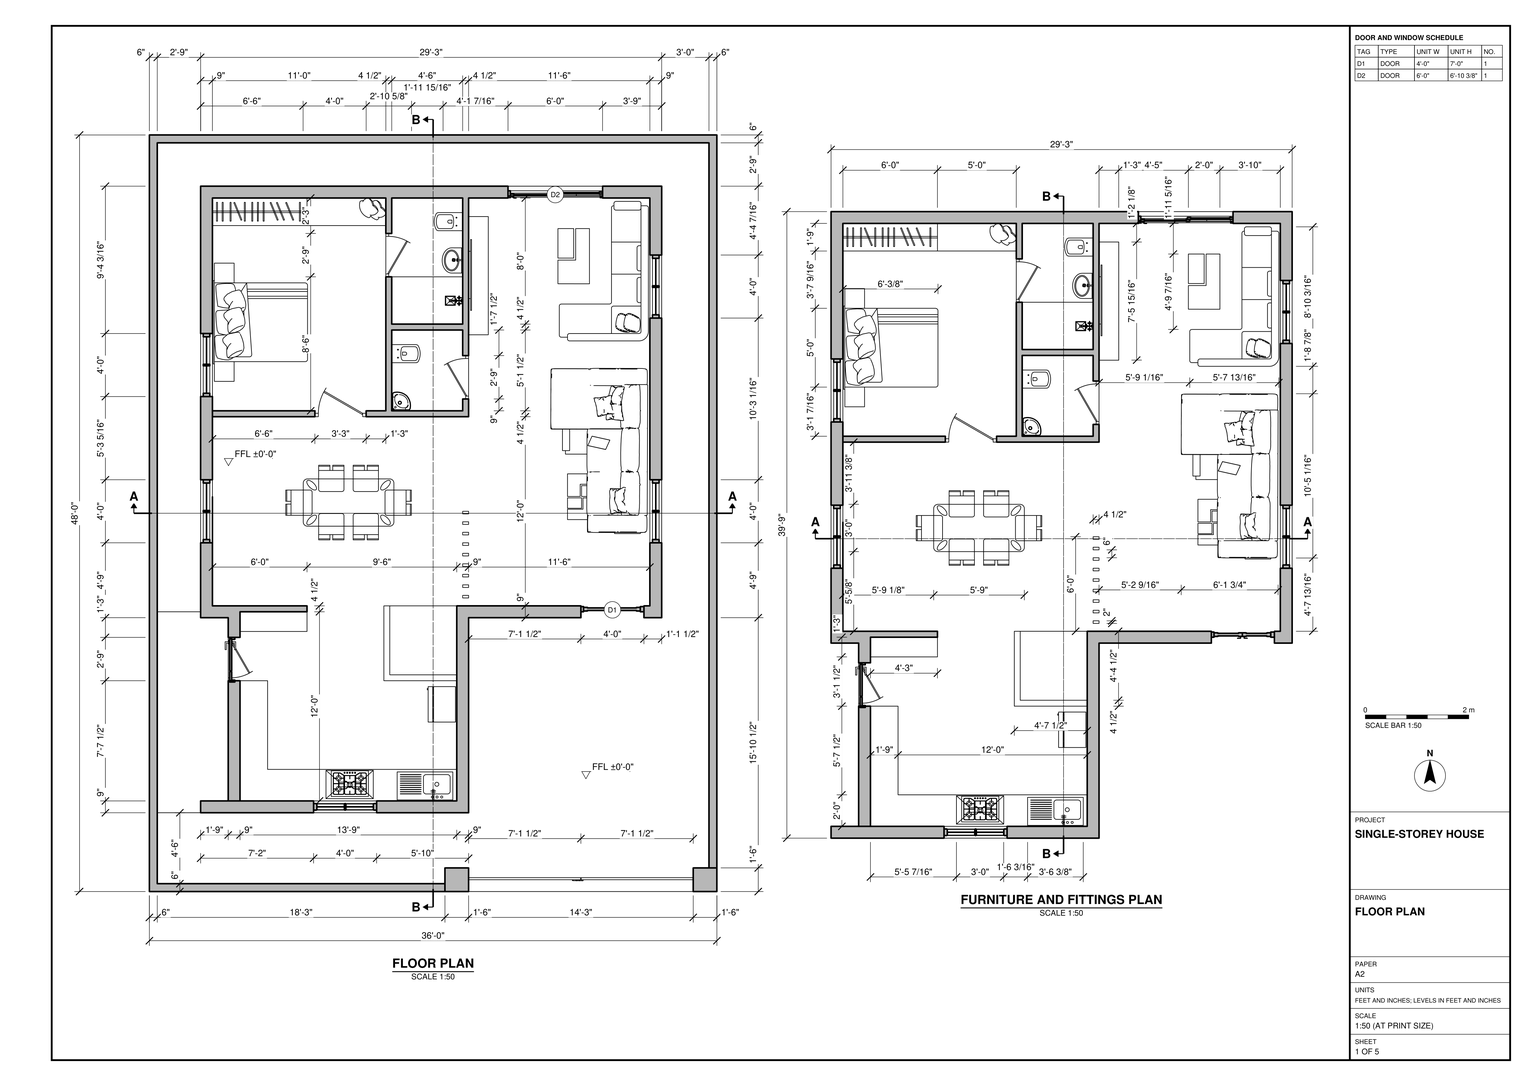
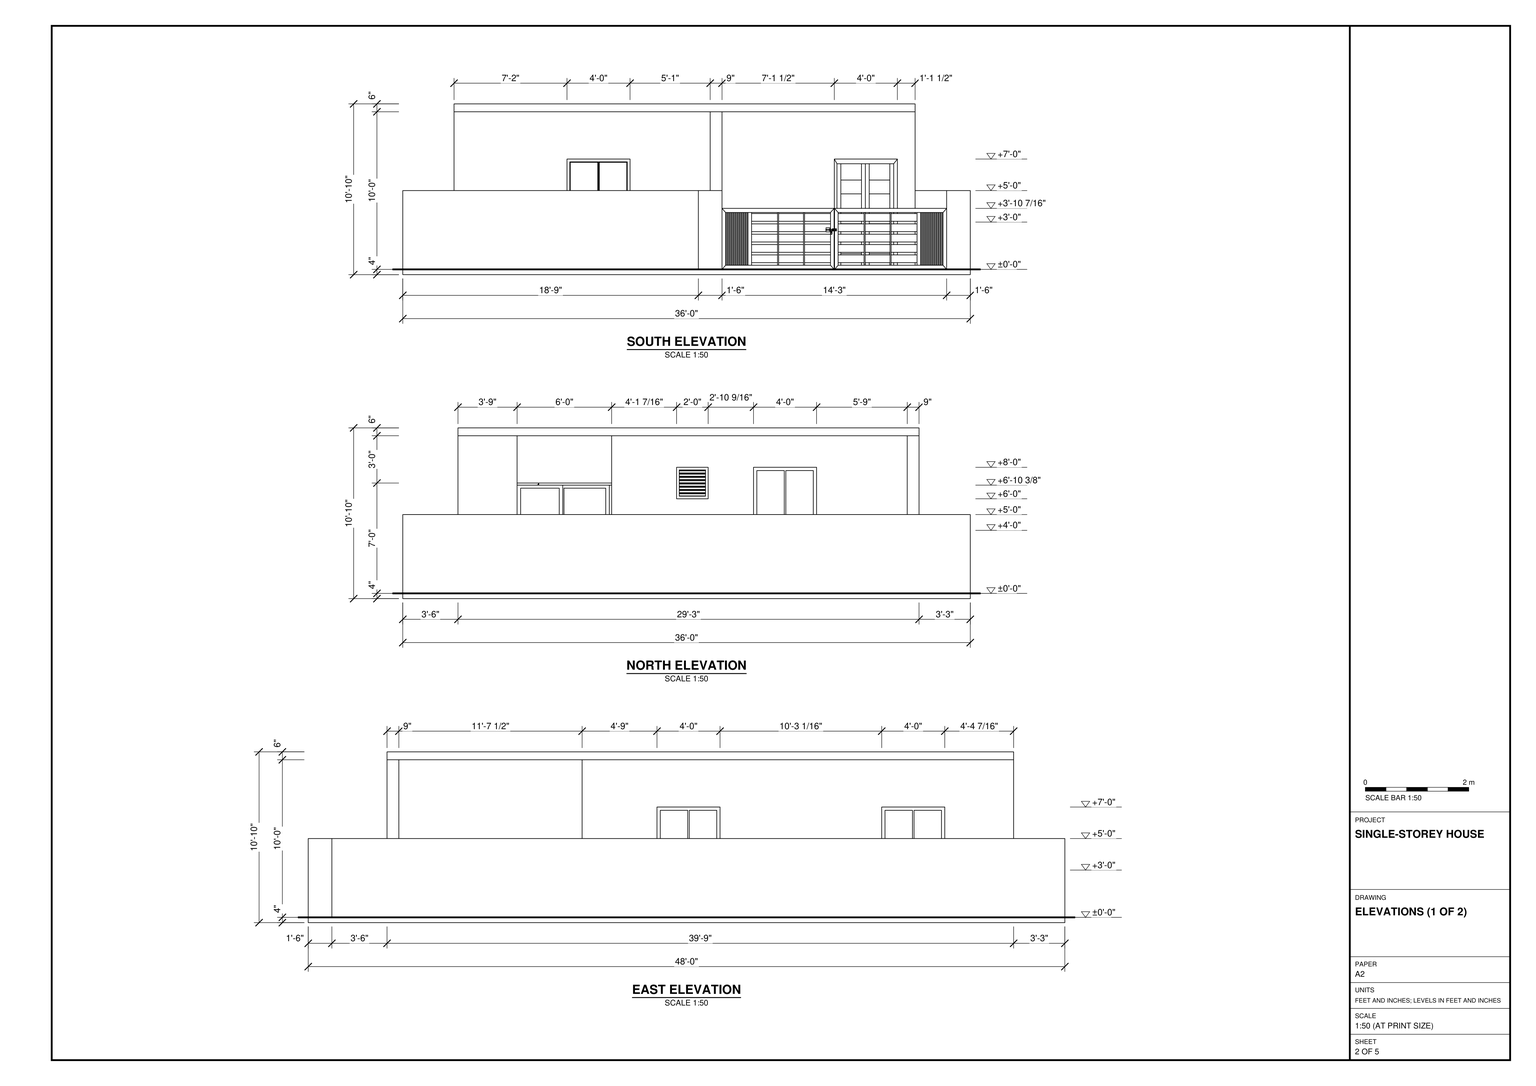
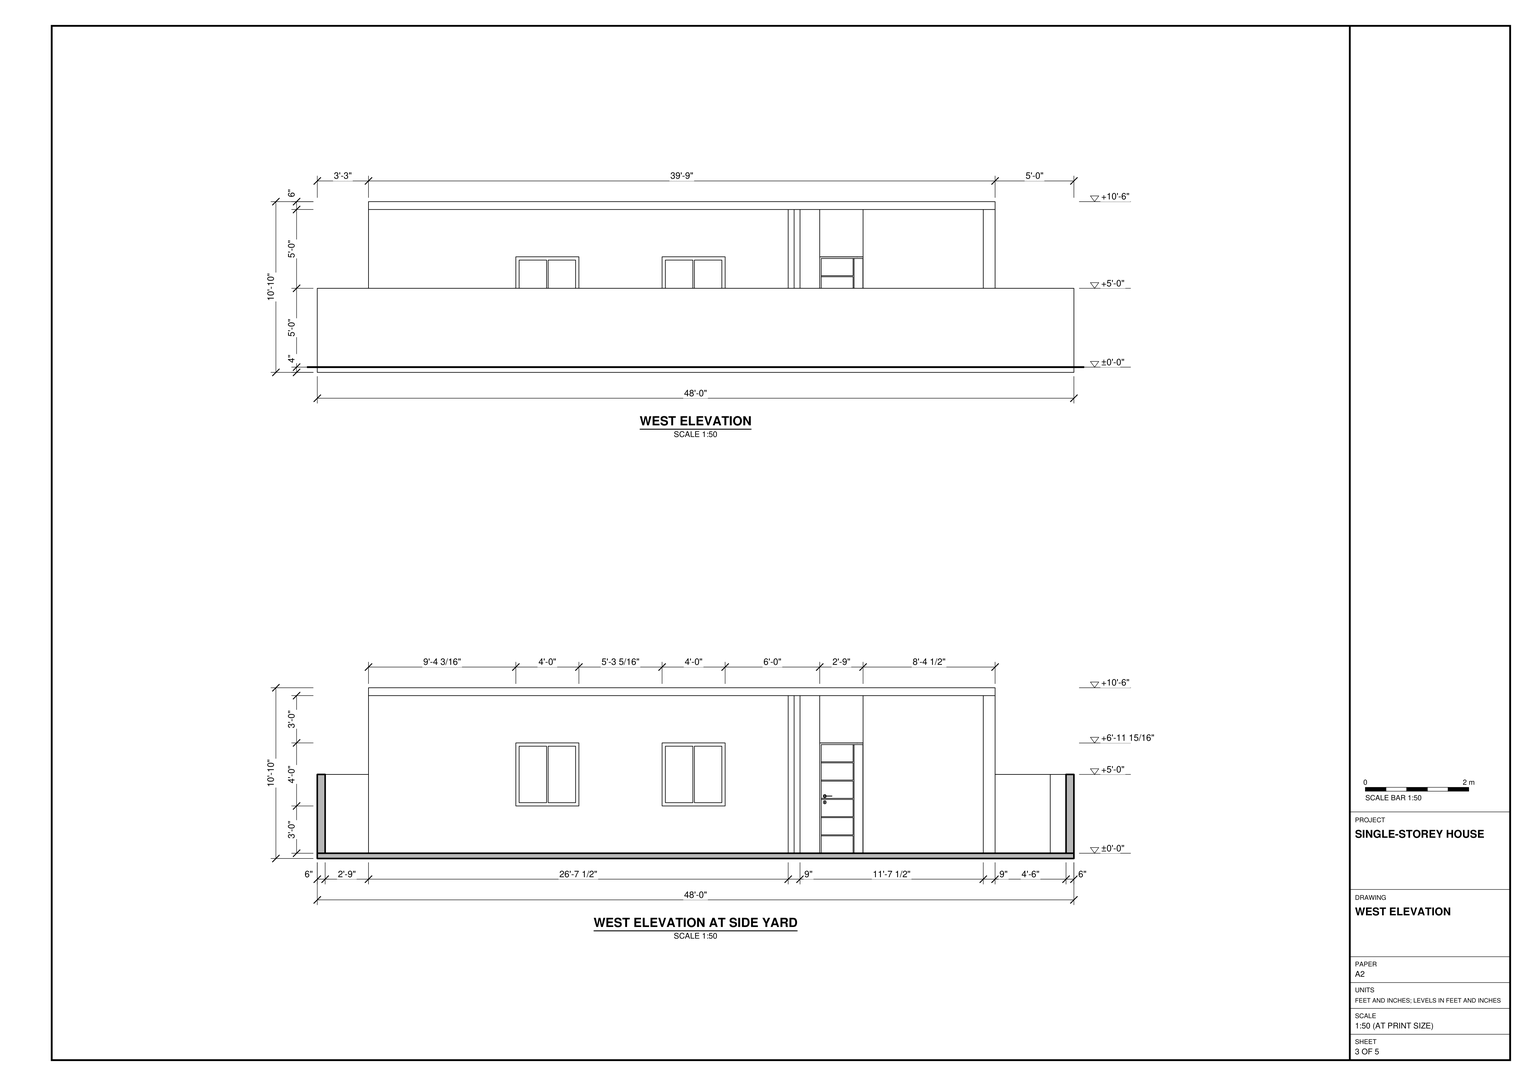
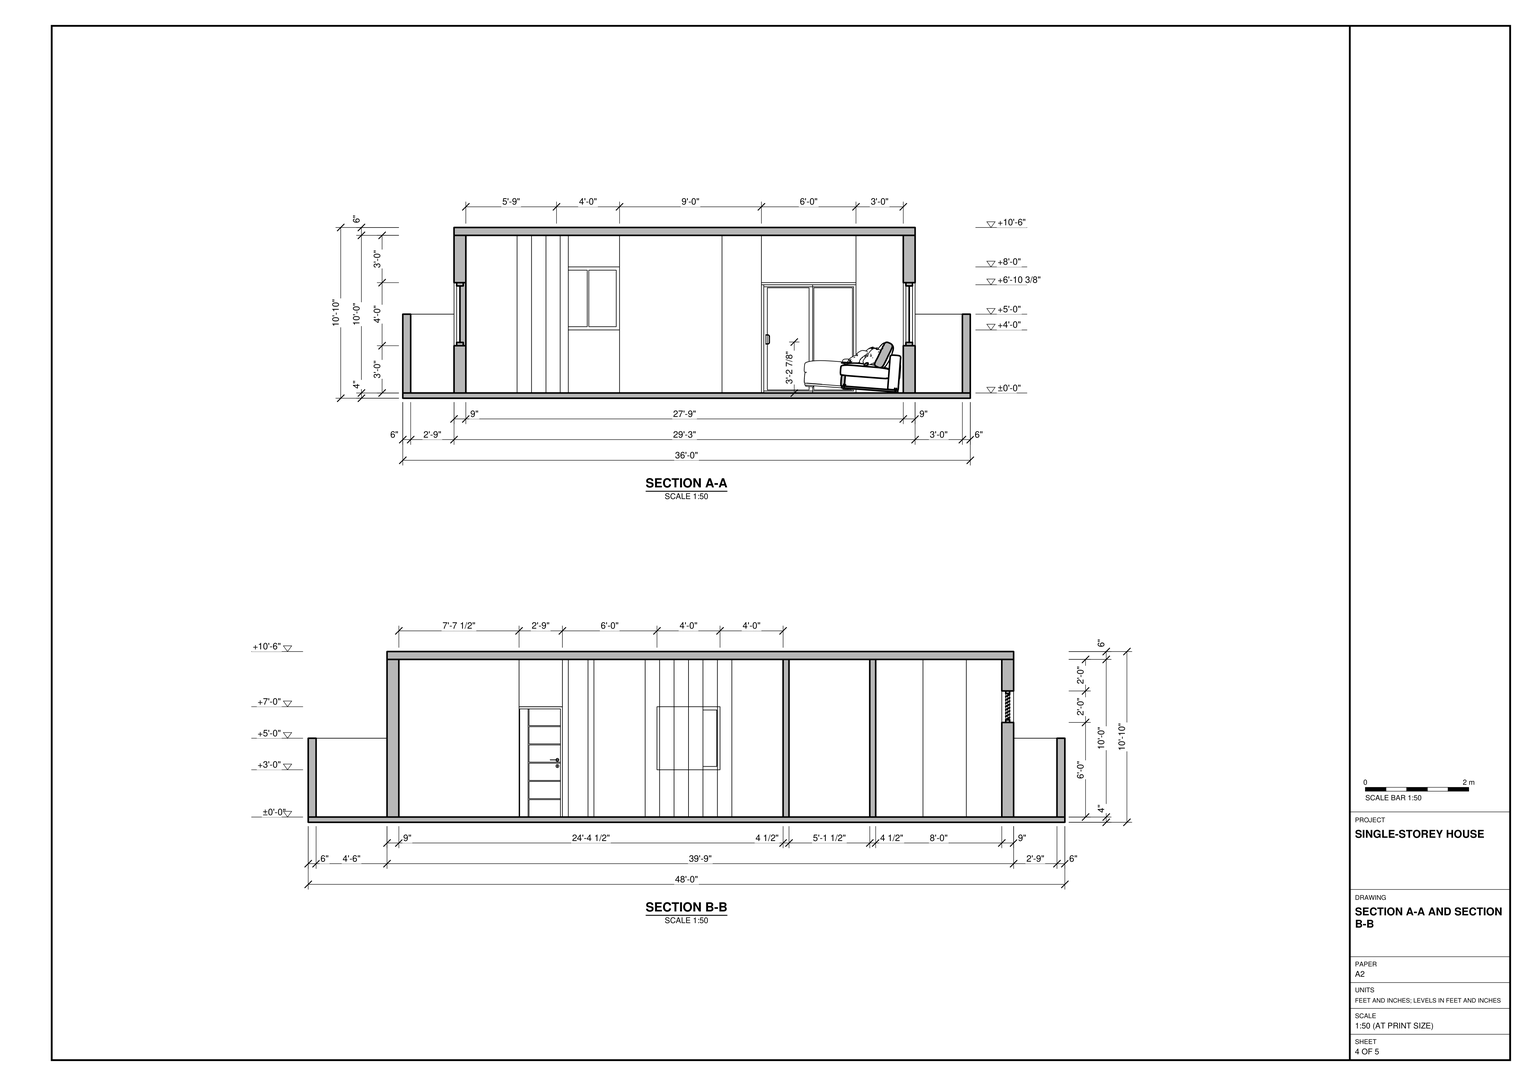
Build the house and its enclosed yard in SketchUp using task_files/diagram_01.pdf. Work in feet and inches. The overall model is 36'-0" east to west, 48'-0" north to south and 10'-10" high, measured from the underside of the ground slab to the top of the flat roof. Set the single finished floor level at ±0'-0".

Use the floor plan to set out the house within the boundary walls. The kitchen projects south from the main block, leaving an entrance yard on its east side. Place the gate between the posts on the south boundary. Model the ground slab, flat roof slab, 9" exterior walls and 4 1/2" interior partitions. Use the elevations and door schedule to locate and size the doors, windows and vent.

Lay out the bedroom in the northwest corner with the bed against the west wall and storage along the north wall. Fit out the two small sanitary rooms beside the bedroom. Follow the furniture and fittings plan for the kitchen counters, sink and cooktop, the dining table and chairs, and the seating and tables on the east side. Match the footprints and orientations shown. Decor and loose items may be any suitable library components.

Keep the walls, slabs and roof separate from one another, and make each furniture or joinery piece a separate group or component. Use components for repeated parts. Save one SketchUp model as output_files/single_storey_house_with_a_gated_yard.skp.

# SketchUp Ruby script. Lengths in inches.
U = 1.inch
M = Sketchup.active_model
def pt(a) = Geom::Point3d.new(a.map { |v| v * U })
def face(e, loops, mat)
  f = e.add_face(loops[0].map { |a| pt(a) })
  loops[1..].each { |l| e.add_face(l.map { |a| pt(a) }).erase! }
  f.material = f.back_material = mat if mat
  f
end
# faces: each face lists its corners as indices into pts; further lists are holes
def faces(e, pts, list, mat = nil) = list.each { |f| face(e, (f[0].is_a?(Array) ? f : [f]).map { |l| l.map { |i| pts[i] } }, mat) }
# xy, xz, yz: faces in a plane at the given z, y or x. An outline is a flat list of corners, or four numbers for a rectangle; further outlines are holes
def ring(l) = l.size == 4 ? [[l[0], l[1]], [l[2], l[1]], [l[2], l[3]], [l[0], l[3]]] : l.each_slice(2).to_a
def flat(e, list, mat, &to3) = list.each { |f| face(e, (f[0].is_a?(Array) ? f : [f]).map { |l| ring(l).map { |u, v| to3.(u, v) } }, mat) }
def xy(e, z, list, mat = nil) = flat(e, list, mat) { |x, y| [x, y, z] }
def xz(e, y, list, mat = nil) = flat(e, list, mat) { |x, z| [x, y, z] }
def yz(e, x, list, mat = nil) = flat(e, list, mat) { |y, z| [x, y, z] }
def lines(e, pts, list) = list.each { |a, b| e.add_line(pt(pts[a]), pt(pts[b])) }
# prism: a flat outline (further loops are holes) pulled along v
def prism(e, loops, v, mat = nil)
  f = face(e, loops, mat); d = Geom::Vector3d.new(v.map { |x| x * U })
  f.pushpull(f.normal.samedirection?(d) ? d.length : -d.length)
end
def box(e, o, s, mat = nil) = prism(e, [[o, [o[0] + s[0], o[1], o[2]], [o[0] + s[0], o[1] + s[1], o[2]], [o[0], o[1] + s[1], o[2]]]], [0, 0, s[2]], mat)
def at(x, y, z, deg = 0) = Geom::Transformation.translation(pt([x, y, z])) * Geom::Transformation.rotation(ORIGIN, Z_AXIS, deg.degrees)
def axes(o, x, y, z) = Geom::Transformation.new([*x, 0, *y, 0, *z, 0, *pt(o).to_a, 1])
def part(name) = M.definitions.add(name)
# library, detail: a bought-in or finely detailed component or shape, given as its bounding box
def library(name, o, s) = part(name).tap { |d| box(d.entities, o, s) }
def detail(e, o, s) = box(e.add_group.entities, o, s)
def put(e, d, t, mat = nil) = e.add_instance(d, t).tap { |i| i.material = mat if mat }
def group(e, t, mat = nil) = e.add_group.tap { |g| g.transformation = t; g.material = mat if mat }.entities
root = M.entities
M.materials.add("0240 AP 7109 IRIS IMPACT").color = [106, 76, 110]
M.materials.add("0250 AP K285 Lilac Linen-N").color = [209, 194, 223]
M.materials.add("0251 AP 9610 Lavender Lyric-N").color = [177, 160, 194]
M.materials.add("[0137_Black]").color = [0, 0, 0]
M.materials.add("[Translucent Glass Blue]").color = [100, 149, 237]
M.materials["[Translucent Glass Blue]"].alpha = 0.5
M.materials.add("[Wood Veneer 01]").color = [120, 70, 37]
c1 = library("SLIDING+GLASS+DOOR",[0,-0.75,0],[72,5.75,80])
c2 = library("RGTE",[-11.95,-7.93,0],[23.9,15.86,0.01])
c3 = part("A$C47E27A62")
p = [[17.04,-15,0],[-17.04,-15,0],[-17.04,-12,0],[17.04,8.51,0],[-17.04,8.51,0],[17.04,15,0],
  [-17.04,15,0],[13.4375,7.07,0],[-13.4375,7.07,0],[-17.04,9.96,0],[-19.5625,9.96,0],[-19.5625,-12,0],
  [-13.4375,-12,0],[-13.4375,8.51,0],[17.04,-12,0],[17.04,9.96,0],[19.5625,9.96,0],[19.5625,-12,0],
  [13.4375,-12,0],[13.4375,8.51,0]]
lines(c3.entities,p,[[0,1],[2,1],[3,4],[5,6],[7,8],[9,10],[6,4],[11,12],[8,12],[13,8],[10,11],[14,0],
  [15,16],[17,18],[19,18],[16,17],[5,3]])
c4 = library("A$C0124305E",[-7.81,-9.6,0],[15.62,19.2,0.01])
c5 = library("RHG",[-21.19,-11.04,0],[42.38,22.08,0.01])
c6 = library("A$Ccaaf8ce0",[-55.9,-35.68,0],[111.8,71.36,0.01])
c7 = library("A$C06e6df2d",[-45.01,-35.89,0],[90.02,71.78,0.01])
c8 = part("A$C338378D9")
p = [[-19.5,-8.5,0],[19.5,-8.5,0],[19.5,15.5,0],[-19.5,15.5,0],[-19.5,-14.5,0],[19.5,-14.5,0],
  [19.5,-9.5,0],[-19.5,-9.5,0],[-18.5,-9.5,0],[-18.5,-8.5,0],[18.5,-9.5,0],[18.5,-8.5,0],
  [-16,-15.5,0],[-17.5,-15.5,0],[-17.5,-14.5,0],[-16,-14.5,0]]
lines(c8.entities,p,[[0,1],[1,2],[2,3],[3,0],[4,5],[5,6],[6,7],[7,4],[8,9],[10,11],[12,13],[13,14],
  [14,15],[15,12]])
c9 = part("A$C08B96C0D")
p = [[18,-10.8,0],[8,-1.8,0],[18,10.8,0],[8,1.8,0],[-18,-10.8,0],[-8,-1.8,0],
  [-18,10.8,0],[-8,1.8,0]]
lines(c9.entities,p,[[0,1],[2,3],[4,5],[6,7],[4,6],[5,7],[1,5],[3,1],[7,3],[0,4],[2,0],[6,2]])
c10 = library("A$C39B3790F",[-21.92,-25.3125,0],[43.84,50.625,0.01])
c11 = part("FHHGGHHJ")
p = [[-7.07,-12.65,0],[-6.44,-13.01,0],[5.93,9.87,0],[5.46,10.12,0],[4.97,10.35,0],[4.49,10.58,0],
  [4,10.8,0],[3.5,11.01,0],[3,11.2,0],[2.5,11.39,0],[1.99,11.57,0],[1.48,11.74,0],
  [0.97,11.89,0],[0.45,12.04,0],[-0.07,12.18,0],[-0.59,12.3,0],[-1.11,12.42,0],[-1.64,12.52,0],
  [-2.17,12.62,0],[-2.7,12.7,0],[-3.23,12.78,0],[-3.76,12.84,0],[-4.3,12.89,0],[-4.83,12.93,0],
  [-5.37,12.96,0],[-5.91,12.98,0],[-6.44,12.99,0],[6.56,9.51,0],[8.43,8.43,0],[-6.43,-13,0],
  [-8.43,-13,0],[-8.43,-15,0],[-6.43,-15,0],[-6.43,15,0],[-8.43,15,0],[-8.43,13,0],
  [-6.43,13,0]]
lines(c11.entities,p,[[0,1],[2,3],[3,4],[4,5],[5,6],[6,7],[7,8],[8,9],[9,10],[10,11],[11,12],[12,13],
  [13,14],[14,15],[15,16],[16,17],[17,18],[18,19],[19,20],[20,21],[21,22],[22,23],[23,24],[24,25],
  [25,26],[27,28],[2,0],[27,2],[1,27],[29,30],[30,31],[31,32],[32,29],[33,34],[34,35],[35,36],
  [36,33]])
c12 = part("A$C0E8E2537")
p = [[30.48,-15,0],[-30.48,-15,0],[-30.48,-12,0],[0,-15,0],[0,7.07,0],[30.48,8.51,0],
  [-30.48,8.51,0],[30.48,15,0],[-30.48,15,0],[26.875,7.07,0],[-26.875,7.07,0],[-30.48,9.96,0],
  [-33,9.96,0],[-33,-12,0],[-26.875,-12,0],[-26.875,8.51,0],[30.48,-12,0],[30.48,9.96,0],
  [33,9.96,0],[33,-12,0],[26.875,-12,0],[26.875,8.51,0]]
lines(c12.entities,p,[[0,1],[2,1],[3,4],[5,6],[7,8],[9,10],[11,12],[8,6],[13,14],[10,14],[15,10],[12,13],
  [16,0],[17,18],[19,20],[21,20],[18,19],[7,5]])
c13 = part("A$C03AA15B9")
p = [[12,-9.82,0],[0,-9.82,0],[0,-0.97,0],[12,-0.97,0],[-1.19,-0.97,0],[-1.19,-10.64,0],
  [12,-10.64,0],[12,-19.5,0],[-12,-19.5,0],[-12,-0.97,0],[-12,9.45,0],[0,9.45,0],
  [0,0.22,0],[-12,0.22,0],[1.19,0.22,0],[1.19,10.64,0],[-12,10.64,0],[-12,19.5,0],
  [12,19.5,0],[12,0.22,0]]
lines(c13.entities,p,[[0,1],[1,2],[2,3],[3,0],[4,5],[5,6],[6,7],[7,8],[8,9],[9,4],[10,11],[11,12],
  [12,13],[13,10],[14,15],[15,16],[16,17],[17,18],[18,19],[19,14]])
c14 = library("A$C7d9d00ca",[-6.89,-10.82,0],[13.78,21.65,0.01])
c15 = part("A$C231C625F")
p = [[-0.375,-18,0],[1.125,-18,0],[1.125,18,0],[-0.375,18,0],[-1.125,-27,0],[-0.375,-27,0],
  [-0.375,27,0],[-1.125,27,0]]
lines(c15.entities,p,[[0,1],[1,2],[2,3],[3,0],[4,5],[5,6],[6,7],[7,4]])
c16 = library("dasd",[-28.43,-47.8125,0],[56.86,95.625,0.01])
c17 = library("A$C4D064DB7",[-6.63,-3.5625,0],[13.26,7.125,0.01])
c18 = part("TABLE 2")
p = [[18.6875,1.33,0],[-2.65,1.33,0],[-2.65,-10.67,0],[-18.65,-10.67,0],[-18.6875,10.67,0],[18.6875,10.67,0],
  [18.6875,0,0],[18.6875,-10.67,0],[-1.28,-10.67,0],[-1.28,0,0]]
lines(c18.entities,p,[[0,1],[1,2],[2,3],[3,4],[4,5],[5,0],[6,7],[7,8],[8,9],[9,6]])
c19 = part("A$C21FE29A1")
p = [[-10,-10,0],[10,-10,0],[10,10,0],[-10,10,0],[-11,-11,0],[11,-11,0],
  [11,11,0],[-11,11,0],[-12,-12,0],[12,-12,0],[12,12,0],[-12,12,0]]
lines(c19.entities,p,[[0,1],[1,2],[2,3],[3,0],[4,5],[5,6],[6,7],[7,4],[8,9],[9,10],[10,11],[11,8]])
c20 = part("dd")
p = [[-6.52,11.67,0],[-5.95,12.01,0],[5.48,-9.11,0],[5.04,-9.34,0],[4.59,-9.56,0],[4.14,-9.77,0],
  [3.6875,-9.97,0],[3.23,-10.16,0],[2.77,-10.34,0],[2.31,-10.52,0],[1.84,-10.68,0],[1.37,-10.83,0],
  [0.89,-10.98,0],[0.42,-11.11,0],[-0.0625,-11.24,0],[-0.54,-11.36,0],[-1.03,-11.46,0],[-1.51,-11.5625,0],
  [-2,-11.65,0],[-2.49,-11.73,0],[-2.98,-11.79,0],[-3.47,-11.85,0],[-3.97,-11.9,0],[-4.46,-11.9375,0],
  [-4.96,-11.97,0],[-5.45,-11.98,0],[-5.95,-11.99,0],[6.05,-8.78,0],[7.79,-7.78,0],[-5.9375,12,0],
  [-7.79,12,0],[-7.79,13.85,0],[-5.9375,13.85,0],[-5.9375,-13.85,0],[-7.79,-13.85,0],[-7.79,-12,0],
  [-5.9375,-12,0]]
lines(c20.entities,p,[[0,1],[2,3],[3,4],[4,5],[5,6],[6,7],[7,8],[8,9],[9,10],[10,11],[11,12],[12,13],
  [13,14],[14,15],[15,16],[16,17],[17,18],[18,19],[19,20],[20,21],[21,22],[22,23],[23,24],[24,25],
  [25,26],[27,28],[2,0],[27,2],[1,27],[29,30],[30,31],[31,32],[32,29],[33,34],[34,35],[35,36],
  [36,33]])
c21 = library("STOVE-3",[-14.15,-9.8,0],[28.3,19.6,0.01])
c22 = library("SH",[-3.77,-3.27,-0.25],[7.54,6.54,0.5])
c23 = part("new bloSDFck")
p = [[-0.99,-2.25,0],[-22.01,-2.25,0],[-0.99,-4.5,0],[-0.99,0,0],[0.99,0,0],[0.99,-4.5,0],
  [-24,-4.5,0],[-24,0,0],[-22.01,0,0],[-22.01,-4.5,0],[22.01,-4.5,0],[22.01,0,0],
  [24,0,0],[24,-4.5,0],[24,4.5,0],[-24,4.5,0],[22.01,-2.25,0],[0.99,-2.25,0]]
lines(c23.entities,p,[[0,1],[2,3],[4,5],[6,7],[7,8],[8,9],[10,11],[11,12],[12,13],[13,6],[13,14],[6,15],
  [15,14],[12,7],[16,17]])
c24 = part("A$C63CB6BFC")
p = [[-24,-4.5,0],[24,-4.5,0],[24,0,0],[-24,0,0],[22.01,2.25,0],[1.02,2.25,0],
  [-0.96,2.25,0],[-22.01,2.25,0],[-0.96,4.5,0],[-0.96,0,0],[1.02,0,0],[1.02,4.5,0],
  [-22.01,0,0],[-22.01,4.5,0],[22.01,0,0],[24,4.5,0],[-24,4.5,0],[22.01,4.5,0]]
lines(c24.entities,p,[[0,1],[2,3],[4,5],[6,7],[8,9],[9,10],[10,11],[3,12],[12,13],[14,2],[15,16],[15,1],
  [16,0],[17,14]])
c25 = part("A$C1F62275E")
p = [[30,-4.5,0],[-30,-4.5,0],[-30,0,0],[30,0,0],[-28.01,2.25,0],[-0.99,2.25,0],
  [0.99,2.25,0],[28.01,2.25,0],[0.99,4.5,0],[0.99,0,0],[-0.99,0,0],[-0.99,4.5,0],
  [28.01,0,0],[28.01,4.5,0],[-28.01,4.5,0],[-28.01,0,0],[-30,4.5,0],[30,4.5,0]]
lines(c25.entities,p,[[0,1],[2,3],[4,5],[6,7],[8,9],[9,10],[10,11],[3,12],[12,13],[14,15],[15,2],[16,17],
  [16,1],[17,0]])
c26 = part("VEN")
p = [[-4.5,-11.98,0],[4.5,-11.98,0],[2.25,10,0],[2.25,-10,0],[0,-11.98,0],[0,11.98,0],
  [0,-10,0],[4.5,-10,0],[4.5,10,0],[0,10,0],[4.5,11.98,0],[-4.5,11.98,0]]
lines(c26.entities,p,[[0,1],[2,3],[4,5],[6,7],[8,9],[1,10],[0,11],[10,11]])
c27 = library("Sectional sofa",[-0.93,-10.63,-23.92],[126.92,88.46,78.25])
c28 = library("PINTU 6 YA",[0,-0.6875,0],[35.83,8.07,80.71])
c29 = library("Double Door",[0,-0.98,0],[62,4.92,84])
c30 = part("Group52\#2")
xy(c30.entities,0,[[-21.5,-21.5,-0.59,21.5],[0.59,-21.5,21.5,21.5]])
c31 = part("Group51\#1")
prism(c31.entities,[[[-24,24,0],[24,24,0],[24,-24,0],[-24,-24,0]],[[0.59,-21.5,0],[21.5,-21.5,0],[21.5,21.5,0],[0.59,21.5,0]],[[-0.59,21.5,0],[-21.5,21.5,0],[-21.5,-21.5,0],[-0.59,-21.5,0]]],[0,0,5])
put(c31.entities,c30,at(0,0,2.5),"[Translucent Glass Blue]")
c32 = part("Group56\#1")
prism(c32.entities,[[[-10,-10,3],[-10,-9.8,3],[-10,-8.07,0],[-10,-8.27,0]]],[20,0,0])
c33 = part("Group57\#1")
prism(c33.entities,[[[10,-7.3,3],[10,-7.5,3],[10,-5.77,0],[10,-5.57,0]]],[-20,0,0])
c34 = part("Group58\#1")
prism(c34.entities,[[[-10,-4.8,3],[-10,-3.07,0],[-10,-3.27,0],[-10,-5,3]]],[20,0,0])
c35 = part("Group59\#1")
prism(c35.entities,[[[10,-0.77,0],[10,-0.57,0],[10,-2.3,3],[10,-2.5,3]]],[-20,0,0])
c36 = part("Group60\#1")
prism(c36.entities,[[[-10,1.73,0],[-10,0,3],[-10,0.2,3],[-10,1.93,0]]],[20,0,0])
c37 = part("Group61\#1")
prism(c37.entities,[[[-10,4.43,0],[-10,4.23,0],[-10,2.5,3],[-10,2.7,3]]],[20,0,0])
c38 = part("Group62\#1")
prism(c38.entities,[[[10,5,3],[10,6.73,0],[10,6.93,0],[10,5.2,3]]],[-20,0,0])
c39 = part("Group63\#1")
prism(c39.entities,[[[10,9.43,0],[10,7.7,3],[10,7.5,3],[10,9.23,0]]],[-20,0,0])
c40 = part("Group54\#1")
put(c40.entities,c32,at(0,0,0))
put(c40.entities,c33,at(0,0,0))
put(c40.entities,c34,at(0,0,0))
put(c40.entities,c35,at(0,0,0))
put(c40.entities,c36,at(0,0,0))
put(c40.entities,c37,at(0,0,0))
put(c40.entities,c38,at(0,0,0))
put(c40.entities,c39,at(0,0,0))
c41 = part("Group64\#2")
xy(c41.entities,0,[[-21.5,-21.5,-0.59,21.5],[0.59,-21.5,21.5,21.5]])
c42 = part("Group63\#2")
prism(c42.entities,[[[24,24,0],[24,-24,0],[-24,-24,0],[-24,24,0]],[[-0.59,21.5,0],[-21.5,21.5,0],[-21.5,-21.5,0],[-0.59,-21.5,0]],[[21.5,-21.5,0],[21.5,21.5,0],[0.59,21.5,0],[0.59,-21.5,0]]],[0,0,5])
put(c42.entities,c41,at(0,0,2.5),"[Translucent Glass Blue]")
c43 = part("Group66\#2")
xy(c43.entities,0,[[-21.5,-21.5,-0.59,21.5],[0.59,-21.5,21.5,21.5]])
c44 = part("Group65\#1")
prism(c44.entities,[[[-24,24,0],[24,24,0],[24,-24,0],[-24,-24,0]],[[0.59,-21.5,0],[21.5,-21.5,0],[21.5,21.5,0],[0.59,21.5,0]],[[-0.59,-21.5,0],[-0.59,21.5,0],[-21.5,21.5,0],[-21.5,-21.5,0]]],[0,0,5])
put(c44.entities,c43,at(0,0,2.5),"[Translucent Glass Blue]")
c45 = part("Group68\#2")
xy(c45.entities,0,[[-21.5,-21.5,-0.59,21.5],[0.59,-21.5,21.5,21.5]])
c46 = part("Group67\#1")
prism(c46.entities,[[[24,24,0],[24,-24,0],[-24,-24,0],[-24,24,0]],[[-21.5,-21.5,0],[-0.59,-21.5,0],[-0.59,21.5,0],[-21.5,21.5,0]],[[0.59,-21.5,0],[21.5,-21.5,0],[21.5,21.5,0],[0.59,21.5,0]]],[0,0,5])
put(c46.entities,c45,at(0,0,2.5),"[Translucent Glass Blue]")
c47 = part("Group70\#2")
xy(c47.entities,0,[[-21.5,-21.5,-0.59,21.5],[0.59,-21.5,21.5,21.5]])
c48 = part("Group69\#1")
prism(c48.entities,[[[24,-24,0],[-24,-24,0],[-24,24,0],[24,24,0]],[[21.5,-21.5,0],[21.5,21.5,0],[0.59,21.5,0],[0.59,-21.5,0]],[[-21.5,21.5,0],[-21.5,-21.5,0],[-0.59,-21.5,0],[-0.59,21.5,0]]],[0,0,5])
put(c48.entities,c47,at(0,0,2.5),"[Translucent Glass Blue]")
c49 = part("Group83\#2")
xy(c49.entities,0,[[-21.5,-21.5,-0.59,21.5],[0.59,-21.5,21.5,21.5]])
c50 = part("Group82\#1")
detail(c50.entities,[-24,-24,0],[48,48,5])
put(c50.entities,c49,at(0,0,2.5),"[Translucent Glass Blue]")
c51 = library("Untitled",[-233.2,-0.83,0],[171,2.4,46.46])
prism(root,[[[126,361.5,4],[119.82,361.5,4],[109,361.5,4],[98,361.5,4],[87,361.5,4],[48,361.5,4],[48,366,4],[126,366,4]]],[0,0,120])
put(root,c1,axes([273,528.5,4],[1,0,0],[0,1,0],[0,0,1.03]))
g1 = group(root,at(-64.99,-89.6,4))
xy(g1,0,[[70.99,149.6,103.99,149.6,103.99,158.6,124.99,158.6,124.99,298.1,103.99,298.1,103.99,302.6,70.99,302.6],[133.99,158.6,298.99,158.6,298.99,182.6,154.99,182.6,154.99,250.1,133.99,250.1],[112.99,596.6,184.99,596.6,184.99,606.5,179.99,606.5,179.99,600.11,179.98,600.1,179.98,600.07,179.97,600.06,179.97,600.05,179.96,600.04,179.95,600.02,179.95,600.01,179.9375,600,179.93,599.99,179.92,599.99,179.89,599.96,179.875,599.96,179.86,599.95,179.85,599.95,179.84,599.94,179.83,599.94,179.8125,599.9375,179.36,599.9375,179.35,599.94,179.34,599.94,179.32,599.95,179.3125,599.95,179.3,599.96,179.29,599.96,179.26,599.99,179.25,599.99,179.22,600.02,179.21,600.04,179.21,600.05,179.2,600.06,179.2,600.07,179.19,600.08,179.19,600.11,179.1875,600.12,179.1875,606.5,172.63,606.5,174.84,601.09,174.84,601.08,174.85,601.07,174.85,600.97,174.84,600.96,174.84,600.9375,174.83,600.92,174.82,600.91,174.82,600.9,174.77,600.85,174.76,600.85,174.75,600.84,174.73,600.83,174.72,600.83,174.35,600.69,174.33,600.6875,174.32,600.6875,174.31,600.68,174.24,600.68,174.23,600.6875,174.21,600.69,174.2,600.7,174.19,600.7,174.18,600.71,174.17,600.71,174.14,600.74,174.125,600.75,174.12,600.76,174.1,600.78,174.1,600.79,174.09,600.81,171.77,606.5,165.59,606.5,167.79,601.09,167.8,601.08,167.8,601.04,167.81,601.03,167.81,601,167.8,600.99,167.8,600.96,167.79,600.95,167.79,600.9375,167.78,600.92,167.78,600.91,167.72,600.85,167.71,600.85,167.7,600.84,167.6875,600.83,167.67,600.83,167.3,600.69,167.29,600.6875,167.27,600.6875,167.26,600.68,167.19,600.68,167.18,600.6875,167.17,600.69,167.16,600.7,167.14,600.7,167.13,600.71,167.12,600.71,167.07,600.76,167.0625,600.77,167.06,600.78,167.05,600.79,167.05,600.81,164.72,606.5,160.79,606.5,162.99,601.09,163,601.08,163,601.04,163.01,601.03,163.01,601,163,600.99,163,600.96,162.99,600.95,162.99,600.9375,162.98,600.92,162.98,600.91,162.92,600.85,162.91,600.85,162.89,600.83,162.875,600.83,162.5,600.69,162.49,600.6875,162.47,600.6875,162.46,600.68,162.39,600.68,162.38,600.6875,162.37,600.69,162.36,600.7,162.34,600.7,162.33,600.71,162.32,600.71,162.26,600.77,162.26,600.78,162.25,600.79,162.25,600.81,159.92,606.5,152.37,606.5,152.37,600.12,152.36,600.11,152.36,600.07,152.35,600.06,152.35,600.05,152.34,600.04,152.33,600.02,152.32,600.01,152.32,600,152.31,599.99,152.3,599.99,152.27,599.96,152.25,599.96,152.24,599.95,152.23,599.95,152.22,599.94,152.21,599.94,152.19,599.9375,151.74,599.9375,151.73,599.94,151.71,599.94,151.7,599.95,151.69,599.95,151.68,599.96,151.67,599.96,151.66,599.97,151.64,599.98,151.63,599.99,151.625,599.99,151.62,600,151.6,600.02,151.59,600.04,151.59,600.05,151.58,600.06,151.58,600.07,151.57,600.08,151.57,606.5,147.93,606.5,147.84,599.9375,147.41,599.9375,147.4,599.94,147.38,599.94,147.37,599.95,147.36,599.95,147.35,599.96,147.34,599.96,147.33,599.97,147.31,599.98,147.27,600.02,147.26,600.04,147.26,600.05,147.25,600.06,147.25,600.07,147.24,600.08,147.24,606.5,143.71,606.5,143.71,600.11,143.7,600.1,143.7,600.07,143.69,600.06,143.6875,600.05,143.68,600.04,143.67,600.02,143.67,600.01,143.65,599.99,143.64,599.99,143.61,599.96,143.6,599.96,143.58,599.95,143.57,599.95,143.56,599.94,143.55,599.94,143.53,599.9375,143.08,599.9375,143.07,599.94,143.06,599.94,143.04,599.95,143.03,599.95,143.02,599.96,143.01,599.96,142.98,599.99,142.97,599.99,142.94,600.02,142.93,600.04,142.93,600.05,142.92,600.06,142.92,600.07,142.91,600.08,142.91,606.5,138.03,606.5,138.03,600.08,138.02,600.07,138.02,600.06,138.01,600.05,138.01,600.04,138,600.02,137.99,600.01,137.99,600,137.98,599.99,137.97,599.99,137.95,599.97,137.93,599.96,137.92,599.96,137.91,599.95,137.9,599.95,137.89,599.94,137.875,599.94,137.86,599.9375,137.41,599.9375,137.4,599.94,137.38,599.94,137.37,599.95,137.36,599.95,137.35,599.96,137.33,599.96,137.32,599.97,137.3125,599.98,137.3,599.99,137.29,599.99,137.28,600,137.28,600.01,137.27,600.02,137.26,600.04,137.26,600.05,137.25,600.06,137.25,600.07,137.24,600.08,137.24,600.12,137.23,600.14,137.23,606.5,133.17,606.5,135.375,601.09,135.38,601.08,135.38,601.05,135.39,601.04,135.39,600.99,135.38,600.97,135.38,600.96,135.375,600.95,135.37,600.9375,135.36,600.92,135.36,600.91,135.32,600.87,135.3125,600.86,135.3,600.85,135.29,600.85,135.27,600.83,135.26,600.83,134.88,600.69,134.87,600.6875,134.86,600.6875,134.84,600.68,134.78,600.68,134.76,600.6875,134.75,600.69,134.74,600.7,134.73,600.7,134.71,600.71,134.7,600.71,134.65,600.76,134.65,600.77,134.63,600.79,134.63,600.81,132.31,606.5,127.19,606.5,127.19,600.11,127.1875,600.1,127.1875,600.08,127.18,600.07,127.18,600.06,127.17,600.05,127.17,600.04,127.16,600.02,127.13,599.99,127.125,599.99,127.11,599.98,127.09,599.96,127.08,599.96,127.07,599.95,127.06,599.95,127.04,599.94,127.03,599.94,127.02,599.9375,126.57,599.9375,126.55,599.94,126.54,599.94,126.53,599.95,126.52,599.95,126.5,599.96,126.49,599.96,126.46,599.99,126.45,599.99,126.43,600.01,126.43,600.02,126.42,600.04,126.41,600.05,126.41,600.06,126.4,600.07,126.4,600.1,126.39,600.11,126.39,606.5,121.19,606.5,121.19,600.1,121.1875,600.08,121.18,600.07,121.18,600.06,121.17,600.05,121.17,600.04,121.16,600.02,121.14,600,121.14,599.99,121.125,599.99,121.12,599.98,121.11,599.97,121.09,599.96,121.08,599.96,121.07,599.95,121.06,599.95,121.05,599.94,121.03,599.94,121.02,599.9375,120.57,599.9375,120.55,599.94,120.54,599.94,120.53,599.95,120.52,599.95,120.51,599.96,120.49,599.96,120.46,599.99,120.45,599.99,120.44,600,120.44,600.01,120.43,600.02,120.42,600.04,120.41,600.05,120.41,600.06,120.4,600.07,120.4,600.11,120.39,600.12,120.39,606.5,116.86,606.5,116.86,600.08,116.85,600.07,116.85,600.06,116.84,600.05,116.84,600.04,116.83,600.02,116.81,600,116.81,599.99,116.8,599.99,116.78,599.97,116.76,599.96,116.75,599.96,116.74,599.95,116.73,599.95,116.72,599.94,116.7,599.94,116.69,599.9375,116.24,599.9375,116.23,599.94,116.21,599.94,116.2,599.95,116.1875,599.95,116.18,599.96,116.16,599.96,116.13,599.99,116.12,599.99,116.11,600,116.11,600.01,116.1,600.02,116.09,600.04,116.08,600.05,116.08,600.06,116.07,600.07,116.07,600.11,116.06,600.12,116.0625,600.14,116.0625,606.5,112.99,606.5],[112.99,606.5,116.0625,607.7],[112.99,607.7,116.0625,607.7,116.0625,614.14,116.06,614.15,116.07,614.16,116.07,614.2,116.08,614.21,116.08,614.22,116.09,614.24,116.11,614.26,116.11,614.27,116.13,614.29,116.14,614.29,116.16,614.31,116.18,614.32,116.1875,614.32,116.2,614.33,116.24,614.33,116.25,614.34,116.68,614.34,116.69,614.33,116.73,614.33,116.74,614.32,116.75,614.32,116.76,614.31,116.78,614.3,116.79,614.29,116.8,614.29,116.81,614.28,116.81,614.27,116.84,614.24,116.84,614.22,116.85,614.21,116.85,614.2,116.86,614.1875,116.86,607.7,120.39,607.7,120.39,614.15,120.4,614.16,120.4,614.2,120.41,614.21,120.41,614.22,120.42,614.24,120.44,614.26,120.44,614.27,120.46,614.29,120.47,614.29,120.49,614.31,120.51,614.32,120.52,614.32,120.53,614.33,120.57,614.33,120.58,614.34,121.01,614.34,121.02,614.33,121.06,614.33,121.07,614.32,121.08,614.32,121.09,614.31,121.11,614.3,121.12,614.29,121.125,614.29,121.14,614.28,121.14,614.27,121.17,614.24,121.17,614.22,121.18,614.21,121.18,614.2,121.1875,614.1875,121.19,614.18,121.19,607.7,126.39,607.7,126.39,614.16,126.4,614.18,126.4,614.2,126.41,614.21,126.41,614.22,126.42,614.24,126.43,614.25,126.43,614.26,126.46,614.29,126.47,614.29,126.5,614.32,126.52,614.32,126.53,614.33,126.57,614.33,126.58,614.34,127.01,614.34,127.02,614.33,127.06,614.33,127.07,614.32,127.08,614.32,127.11,614.29,127.125,614.29,127.13,614.28,127.17,614.24,127.17,614.22,127.18,614.21,127.18,614.2,127.1875,614.1875,127.1875,614.18,127.19,614.16,127.19,607.7,131.82,607.7,129.31,613.87,129.3,613.88,129.3,613.9,129.29,613.91,129.29,613.98,129.3,613.99,129.3,614.01,129.31,614.03,129.3125,614.04,129.32,614.05,129.33,614.0625,129.34,614.07,129.34,614.08,129.36,614.1,129.39,614.12,129.4,614.12,129.41,614.13,129.42,614.13,129.8,614.27,129.8125,614.27,129.82,614.28,129.92,614.28,129.93,614.27,129.94,614.27,129.95,614.26,129.97,614.26,130.03,614.2,130.03,614.19,130.05,614.17,130.05,614.16,132.68,607.7,137.23,607.7,137.23,614.14,137.24,614.15,137.24,614.1875,137.25,614.2,137.25,614.21,137.26,614.22,137.26,614.24,137.28,614.26,137.28,614.27,137.3,614.29,137.3125,614.29,137.32,614.3,137.33,614.31,137.35,614.32,137.36,614.32,137.37,614.33,137.41,614.33,137.42,614.34,137.85,614.34,137.86,614.33,137.9,614.33,137.91,614.32,137.92,614.32,137.93,614.31,137.95,614.3,137.96,614.29,137.97,614.29,137.99,614.27,137.99,614.26,138.01,614.24,138.01,614.22,138.02,614.21,138.02,614.2,138.03,614.1875,138.03,607.7,142.91,607.7,142.91,614.1875,142.92,614.2,142.92,614.21,142.93,614.22,142.93,614.24,142.98,614.29,142.99,614.29,143.02,614.32,143.03,614.32,143.04,614.33,143.08,614.33,143.09,614.34,143.52,614.34,143.53,614.33,143.57,614.33,143.58,614.32,143.6,614.32,143.63,614.29,143.64,614.29,143.67,614.26,143.67,614.25,143.68,614.24,143.6875,614.22,143.69,614.21,143.7,614.2,143.7,614.18,143.71,614.16,143.71,607.7,147.24,607.7,147.24,614.1875,147.25,614.2,147.25,614.21,147.26,614.22,147.26,614.24,147.3,614.28,147.3,614.29,147.31,614.29,147.33,614.3,147.35,614.32,147.36,614.32,147.37,614.33,147.41,614.33,147.42,614.34,147.85,614.34,147.86,614.33,147.9,614.33,147.91,614.32,147.93,614.32,147.9375,614.31,147.95,614.3,147.96,614.29,147.97,614.29,148,614.26,148,614.25,148.01,614.24,148.02,614.22,148.02,614.21,148.03,614.2,148.03,614.16,148.04,614.15,148.04,614.14,147.95,607.7,151.57,607.7,151.57,614.1875,151.58,614.2,151.58,614.21,151.59,614.22,151.59,614.24,151.62,614.27,151.63,614.29,151.64,614.29,151.66,614.3,151.68,614.32,151.69,614.32,151.7,614.33,151.74,614.33,151.75,614.34,152.18,614.34,152.19,614.33,152.23,614.33,152.24,614.32,152.25,614.32,152.27,614.31,152.29,614.29,152.3,614.29,152.32,614.27,152.32,614.26,152.34,614.24,152.35,614.22,152.35,614.21,152.36,614.2,152.36,614.16,152.37,614.15,152.37,607.7,159.4375,607.7,156.92,613.87,156.92,613.9,156.91,613.91,156.91,613.99,156.92,614,156.92,614.01,156.93,614.03,156.93,614.04,156.9375,614.05,156.95,614.0625,156.95,614.07,157,614.12,157.02,614.12,157.03,614.13,157.04,614.13,157.42,614.27,157.43,614.27,157.44,614.28,157.53,614.28,157.55,614.27,157.56,614.27,157.57,614.26,157.58,614.26,157.6,614.25,157.62,614.23,157.625,614.22,157.64,614.21,157.64,614.2,157.66,614.18,157.66,614.17,157.67,614.16,160.3,607.7,164.24,607.7,161.72,613.87,161.72,613.9,161.71,613.91,161.71,613.99,161.72,614,161.72,614.01,161.73,614.03,161.73,614.04,161.74,614.05,161.75,614.0625,161.75,614.07,161.8,614.12,161.82,614.12,161.83,614.13,161.84,614.13,162.22,614.27,162.23,614.27,162.24,614.28,162.33,614.28,162.35,614.27,162.36,614.27,162.37,614.26,162.38,614.26,162.4,614.25,162.44,614.21,162.44,614.2,162.46,614.18,162.46,614.17,162.47,614.16,165.1,607.7,171.28,607.7,168.77,613.87,168.77,613.88,168.76,613.9,168.76,614,168.77,614.01,168.77,614.03,168.79,614.05,168.79,614.0625,168.8,614.07,168.85,614.12,168.86,614.12,168.875,614.13,168.89,614.13,169.26,614.27,169.28,614.27,169.29,614.28,169.38,614.28,169.39,614.27,169.41,614.27,169.42,614.26,169.43,614.26,169.5,614.19,169.5,614.18,169.52,614.16,172.15,607.7,179.1875,607.7,179.1875,614.15,179.19,614.16,179.19,614.1875,179.2,614.2,179.2,614.21,179.21,614.22,179.21,614.24,179.26,614.29,179.27,614.29,179.3,614.32,179.3125,614.32,179.32,614.33,179.36,614.33,179.375,614.34,179.8,614.34,179.8125,614.33,179.85,614.33,179.86,614.32,179.875,614.32,179.89,614.31,179.91,614.29,179.92,614.29,179.93,614.28,179.9375,614.27,179.95,614.26,179.95,614.25,179.96,614.24,179.97,614.22,179.97,614.21,179.98,614.2,179.98,614.18,179.99,614.16,179.99,607.7,184.99,607.7,184.99,617.6,112.99,617.6]])
# 156 loose lines left out
put(g1,c2,axes([234.92,609.22,0],[-0.86556,0.2466,0],[-0.2466,-0.86556,0],[0,0,0.9]))
put(g1,c3,axes([396.92,436,0],[0.89319,0,0],[0,0.89319,0],[0,0,0.89319]))
put(g1,c4,at(295.68,570.06,0))
put(g1,c5,axes([274.8,169.64,0],[1,0,0],[0,-1,0],[0,0,1]))
put(g1,c6,axes([410.95,561.92,0],[0,-0.95,0],[-0.95,0,0],[0,0,0.95]))
put(g1,c7,at(149.48,523.01,0,-90))
put(g1,c8,axes([287.24,232.13,0],[0,-0.69231,0],[0.69231,0,0],[0,0,0.69231]))
put(g1,c9,axes([217.43,171.1,0],[1,0,0],[0,-1,0],[0,0,1]))
put(g1,c10,axes([255.51,461.6,0],[-0.2514,-0.2514,0],[0.2514,-0.2514,0],[0,0,0.35554]))
put(g1,c11,axes([298.71,481.1,0],[-1.1,0,0],[0,1.1,0],[0,0,1.1]))
put(g1,c12,axes([429.83,391.58,0],[0,0.89319,0],[0.89319,0,0],[0,0,0.89319]))
put(g1,c11,axes([254.27,574.1,0],[1.1,0,0],[0,1.1,0],[0,0,1.1]))
put(g1,c13,axes([394,390.18,0],[-0.89319,0,0],[0,0.89319,0],[0,0,0.89319]))
put(g1,c14,at(292.66,599.6,0,-90))
put(g1,c15,axes([309.11,559.02,0],[-1,0,0],[0,1,0],[0,0,1]))
put(g1,c16,at(216.62,385.76,0,-90))
put(g1,c17,axes([296.85,539.41,0],[1,0,0],[0,-1,0],[0,0,1]))
put(g1,c18,axes([388.01,573.3,0],[0,1.125,0],[1.125,0,0],[0,0,1.125]))
put(g1,c19,axes([429.06,435.56,0],[0,-0.89319,0],[0.89319,0,0],[0,0,0.89319]))
put(g1,c20,axes([210.49,462.07,0],[0,1.40833,0],[1.40833,0,0],[0,0,1.40833]))
put(g1,c21,axes([217.57,171.76,0],[-1,0,0],[0,1,0],[0,0,1]))
put(g1,c11,axes([134.27,266.6,0],[1.1,0,0],[0,-1.1,0],[0,0,1.1]))
put(g1,c22,axes([300.21,539.38,0.25],[0,1.00172,0],[1.00172,0,0],[0,0,1.00172]))
put(g1,c14,axes([260.32,499.1,0],[0,-1,0],[-1,0,0],[0,0,1]))
put(g1,c23,at(108.49,379.1,0,90))
put(g1,c24,axes([450.49,550.18,0],[0,-1,0],[-1,0,0],[0,0,1]))
put(g1,c24,axes([205.99,622.1,0],[1,0,0],[0,-1,0],[0,0,1]))
put(g1,c24,axes([450.49,379.1,0],[0,-1,0],[-1,0,0],[0,0,1]))
put(g1,c25,at(219.99,154.1,0))
put(g1,c24,axes([108.49,490.44,0],[0,1,0],[1,0,0],[0,0,1]))
put(g1,c26,at(276.57,622.1,0,-90))
put(g1,c27,axes([443.23,362.9,1.375],[0,1,0],[-0.99706,0,0.07661],[0.07661,0,0.99706]))
g2 = group(root,at(39,60,4),"0251 AP 9610 Lavender Lyric-N")
xy(g2,0,[[0,0,204,9],[337.5,148.5,351,157.5]])
xy(g2,36,[[86,0,134,4.5],[86,4.5,134,9],[0,205.5,4.5,253.5],[4.5,205.5,9,253.5],[342,205.5,346.5,253.5],
  [346.5,205.5,351,253.5],[0,316.84,4.5,364.84],[4.5,316.84,9,364.84],[342,376.58,346.5,424.58],[346.5,376.58,351,424.58]])
xy(g2,48,[[78,468,126,472.5],[78,472.5,126,477]])
xy(g2,72,[[160.56,468,184.56,472.5],[160.56,472.5,184.56,477]])
xy(g2,84,[[86,0,134,4.5],[86,4.5,134,9],[21,100.5,30,133.5],[289.5,148.5,337.5,157.5],[0,205.5,4.5,253.5],
  [4.5,205.5,9,253.5],[342,205.5,346.5,253.5],[346.5,205.5,351,253.5],[0,316.84,4.5,364.84],[4.5,316.84,9,364.84],
  [342,376.58,346.5,424.58],[346.5,376.58,351,424.58],[234,468,306,477]])
xy(g2,96,[[78,468,126,472.5],[160.56,468,184.56,472.5],[78,472.5,126,477],[160.56,472.5,184.56,477]])
xy(g2,120,[[0,0,204,9],[21,9,30,100.5],[195,9,204,9,204,148.5,351,148.5,351,477,306,477,306,468,342,468,342,157.5,195,157.5],[21,133.5,30,133.5,30,153,81,153,81,157.5,9,157.5,9,148.5,21,148.5],[0,148.5,9,157.5],
  [0,157.5,9,477],[126,301.5,204,301.5,204,315,199.5,315,199.5,306,145.5,306,145.5,367.5,199.5,367.5,199.5,348,204,348,204,468,234,468,234,477,9,477,9,468,141,468,141,441,145.5,441,145.5,468,199.5,468,199.5,372,145.5,372,145.5,408,141,408,141,306,126,306],[234,468,306,477]])
xz(g2,0,[[[0,0,195,120],[86,36,134,84]],[195,0,204,120]])
xz(g2,9,[[0,0,21,120],[21,0,30,120],[[30,0,195,120],[86,36,134,84]]])
xz(g2,100.5,[[21,0,30,84],[21,84,30,120]])
xz(g2,133.5,[[21,0,30,84],[21,84,30,120]])
xz(g2,148.5,[[0,0,9,120],[9,0,21,120],[204,0,289.5,0,289.5,84,337.5,84,337.5,0,351,0,351,120,204,120]])
xz(g2,153,[[30,0,81,120]])
xz(g2,157.5,[[9,0,48,120],[48,0,59,120],[59,0,70,120],[70,0,81,120],[195,0,289.5,120],
  [337.5,0,342,120],[289.5,84,337.5,120]])
xz(g2,205.5,[[0,36,4.5,84],[4.5,36,9,84],[342,36,346.5,84],[346.5,36,351,84]])
xz(g2,253.5,[[0,36,4.5,84],[4.5,36,9,84],[342,36,346.5,84],[346.5,36,351,84]])
xz(g2,301.5,[[126,0,204,120]])
xz(g2,306,[[126,0,141,120],[145.5,0,199.5,120]])
xz(g2,315,[[199.5,0,204,120]])
xz(g2,316.84,[[0,36,4.5,84],[4.5,36,9,84]])
xz(g2,348,[[199.5,0,204,120]])
xz(g2,364.84,[[0,36,4.5,84],[4.5,36,9,84]])
xz(g2,367.5,[[145.5,0,199.5,120]])
xz(g2,372,[[145.5,0,199.5,120]])
xz(g2,376.58,[[342,36,346.5,84],[346.5,36,351,84]])
xz(g2,408,[[141,0,145.5,120]])
xz(g2,424.58,[[342,36,346.5,84],[346.5,36,351,84]])
xz(g2,441,[[141,0,145.5,120]])
xz(g2,468,[[9,0,81,0,81,48,78,48,78,96,81,96,81,120,9,120],[81,0,141,0,141,120,81,120,81,96,126,96,126,48,81,48],[[145.5,0,199.5,120],[160.56,72,184.56,96]],[204,0,234,120],[306,0,342,120],
  [78,48,81,96],[234,84,306,120]])
xz(g2,477,[[0,0,9,120],[[9,0,234,120],[78,48,126,96],[160.56,72,184.56,96]],[306,0,351,120],[234,84,306,120]])
yz(g2,0,[[0,0,9,120],[148.5,0,153,120],[153,0,157.5,120],[[157.5,0,477,120],[316.84,36,364.84,84],[205.5,36,253.5,84]]])
yz(g2,9,[[157.5,0,196.5,120],[196.5,0,207.5,0,207.5,36,205.5,36,205.5,84,207.5,84,207.5,120,196.5,120],[207.5,0,218.5,36],[218.5,0,229.5,36],[229.5,0,240.5,36],
  [240.5,0,251.5,36],[251.5,0,262.5,0,262.5,120,251.5,120,251.5,84,253.5,84,253.5,36,251.5,36],[262.5,0,301.5,120],[301.5,0,306,120],[[306,0,447,120],[316.84,36,364.84,84]],
  [447,0,456.9,120],[456.9,0,458.1,120],[458.1,0,468,120],[205.5,36,207.5,84],[207.5,36,218.5,84],
  [218.5,36,229.5,84],[229.5,36,240.5,84],[207.5,84,218.5,120],[218.5,84,229.5,120],[229.5,84,240.5,120],
  [240.5,84,251.5,120]])
yz(g2,21,[[9,0,100.5,120],[133.5,0,148.5,120],[100.5,84,133.5,120]])
yz(g2,30,[[9,0,100.5,120],[133.5,0,138,120],[138,0,153,120],[100.5,84,133.5,120]])
yz(g2,78,[[468,48,472.5,96],[472.5,48,477,96]])
yz(g2,81,[[153,0,157.5,120]])
yz(g2,86,[[0,36,4.5,84],[4.5,36,9,84]])
yz(g2,126,[[301.5,0,304.1,120],[304.1,0,306,120],[468,48,472.5,96],[472.5,48,477,96]])
yz(g2,134,[[0,36,4.5,84],[4.5,36,9,84]])
yz(g2,141,[[306,0,408,120],[441,0,447,120],[447,0,468,120]])
yz(g2,145.5,[[306,0,367.5,120],[372,0,408,120],[441,0,468,120]])
yz(g2,160.56,[[468,72,472.5,96],[472.5,72,477,96]])
yz(g2,184.56,[[468,72,472.5,96],[472.5,72,477,96]])
yz(g2,195,[[9,0,33,120],[33,0,100.5,120],[100.5,0,105,120],[105,0,157.5,120]])
yz(g2,199.5,[[306,0,315,120],[348,0,367.5,120],[372,0,408,120],[408,0,468,120]])
yz(g2,204,[[0,0,9,120],[9,0,148.5,120],[301.5,0,315,120],[348,0,363.86,120],[363.86,0,453.86,120],
  [453.86,0,468,120]])
yz(g2,234,[[468,0,473.5,84],[473.5,0,477,84],[468,84,473.5,120],[473.5,84,477,120]])
yz(g2,289.5,[[148.5,0,157.5,84]])
yz(g2,306,[[468,0,473.5,84],[473.5,0,477,84],[468,84,473.5,120],[473.5,84,477,120]])
yz(g2,337.5,[[148.5,0,157.5,84]])
yz(g2,342,[[[157.5,0,468,120],[205.5,36,253.5,84],[376.58,36,424.58,84]]])
yz(g2,351,[[[148.5,0,477,120],[205.5,36,253.5,84],[376.58,36,424.58,84]]])
# 2 loose lines left out
put(g2,c28,axes([26.04,133.5,0],[0,-0.94865,0],[-1,0,0],[0,0,1.04]))
put(g2,c29,axes([289.5,153,0],[0.77419,0,0],[0,1,0],[0,0,1]))
put(g2,c31,axes([102,470,72],[-1,0,0],[0,0,1],[0,1,0]),"[Wood Veneer 01]")
g3 = group(g2,at(160.56,472.5,72))
xy(g3,0,[[0,-1.5,24,1.5]],"[0137_Black]")
xy(g3,2,[[2,-1.5,22,0],[2,0,22,1.5]],"[0137_Black]")
xy(g3,22,[[2,-1.5,22,0],[2,0,22,1.5]],"[0137_Black]")
xy(g3,24,[[0,-1.5,24,1.5]],"[0137_Black]")
xz(g3,-1.5,[[[0,0,24,24],[2,2,22,22]]],"[0137_Black]")
xz(g3,1.5,[[[0,0,24,24],[2,2,22,22]]],"[0137_Black]")
yz(g3,0,[[-1.5,0,1.5,24]],"[0137_Black]")
yz(g3,2,[[-1.5,2,0,22],[0,2,1.5,22]],"[0137_Black]")
yz(g3,22,[[-1.5,2,0,22],[0,2,1.5,22]],"[0137_Black]")
yz(g3,24,[[-1.5,0,1.5,24]],"[0137_Black]")
put(g3,c40,axes([12,1.5,12],[1,0,0],[0,0,1],[0,-1,0]))
put(g2,c42,axes([344,400.58,60],[0,1,0],[0,0,1],[1,0,0]),"[Wood Veneer 01]")
put(g2,c44,axes([344,229.5,60],[0,1,0],[0,0,1],[1,0,0]),"[Wood Veneer 01]")
put(g2,c46,axes([7,340.84,60],[0,-1,0],[0,0,1],[-1,0,0]),"[Wood Veneer 01]")
put(g2,c48,axes([7,229.5,60],[0,-1,0],[0,0,1],[-1,0,0]),"[Wood Veneer 01]")
put(g2,c50,axes([110,7,60],[1,0,0],[0,0,1],[0,-1,0]),"[Wood Veneer 01]")
g4 = group(root,at(39,60,124),"0240 AP 7109 IRIS IMPACT")
box(g4,[0,0,0],[351,477,6])
g5 = group(root,at(6,18,4),"0250 AP K285 Lilac Linen-N")
prism(g5,[[[426,558,0],[426,0,0],[420,0,0],[420,552,0],[0,552,0],[0,-12,0],[219,-12,0],[219,-18,0],[-6,-18,0],[-6,558,0]]],[0,0,60])
g6 = group(root,at(0,0,4))
xy(g6,-4,[[0,0,432,576]])
xy(g6,0,[[0,0,225,0,225,18,243,18,243,0,414,0,414,18,432,18,432,576,0,576]])
xy(g6,60,[[225,0,243,18],[414,0,432,18]])
xz(g6,0,[[0,-4,432,-4,432,60,414,60,414,0,243,0,243,60,225,60,225,0,0,0]])
xz(g6,18,[[225,0,243,60],[414,0,432,60]])
xz(g6,576,[[0,-4,432,0]])
yz(g6,0,[[0,-4,576,0]])
yz(g6,225,[[0,0,18,60]])
yz(g6,243,[[0,0,18,60]])
yz(g6,414,[[0,0,18,60]])
yz(g6,432,[[0,-4,576,-4,576,0,18,0,18,60,0,60]])
put(g6,c51,at(476.2,9,0))
